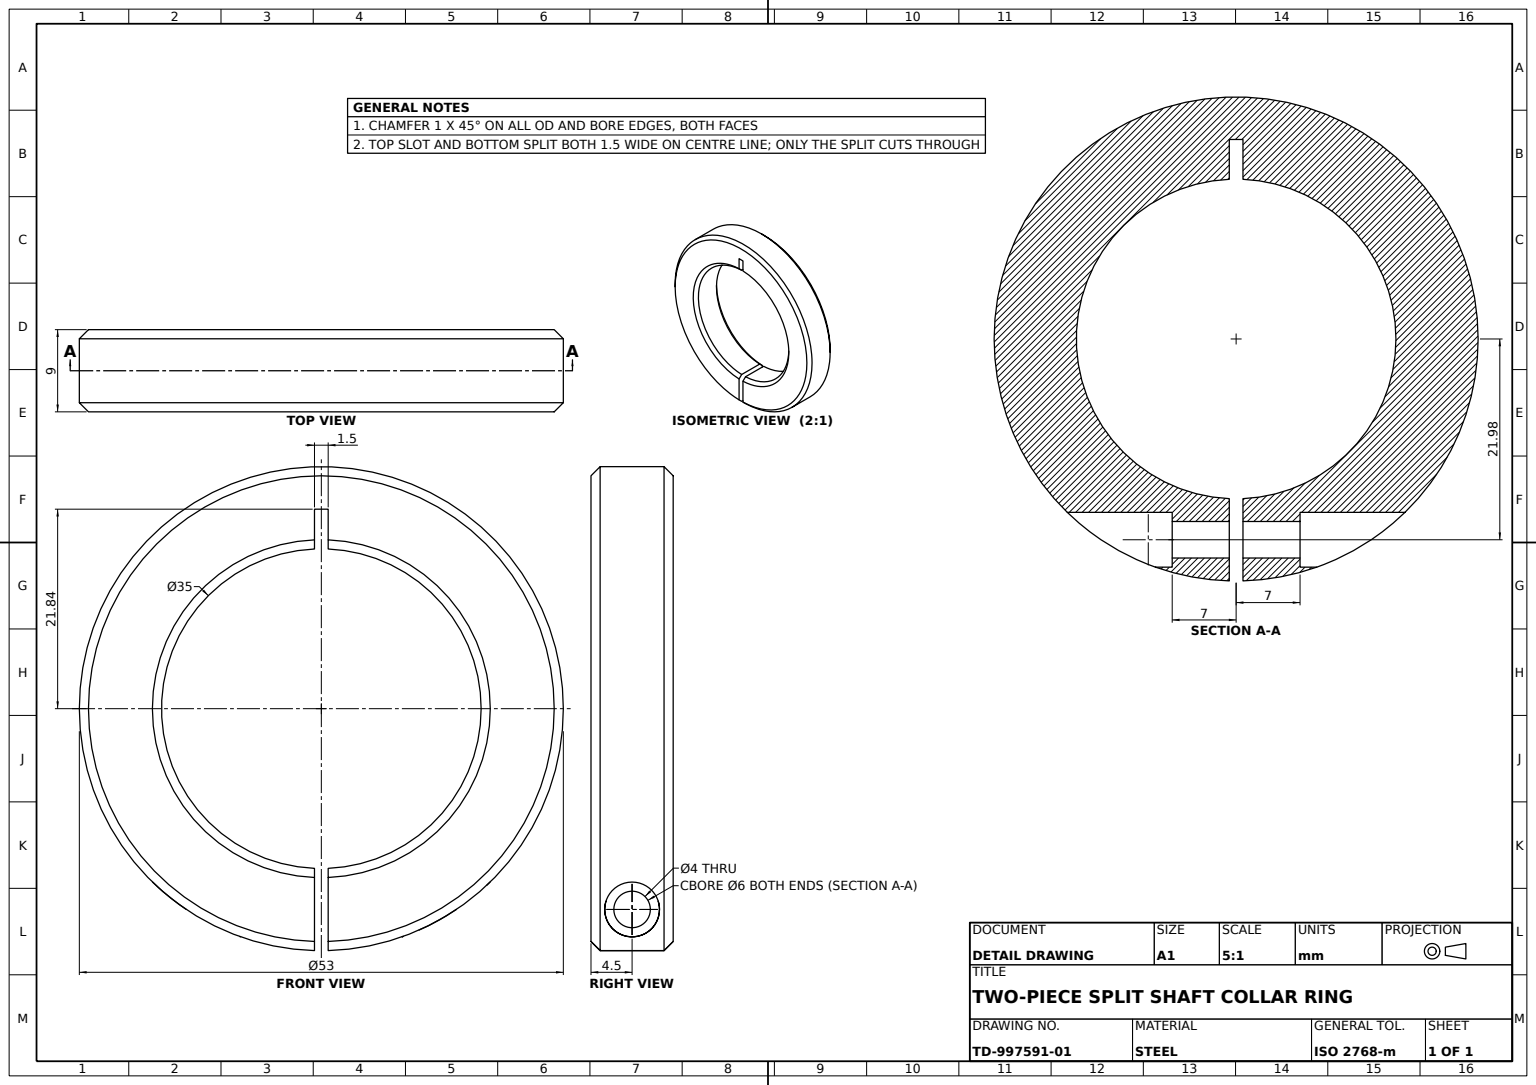
ISO-10303-21;
HEADER;
FILE_DESCRIPTION((''),'2;1');
FILE_NAME('','',(''),(''),'','','');
FILE_SCHEMA(('AUTOMOTIVE_DESIGN'));
ENDSEC;
DATA;
#1=APPLICATION_CONTEXT('');
#2=PRODUCT_CONTEXT('',#1,'mechanical');
#3=PRODUCT('','','',(#2));
#4=PRODUCT_DEFINITION_FORMATION('','',#3);
#5=PRODUCT_DEFINITION_CONTEXT('',#1,'design');
#6=PRODUCT_DEFINITION('','',#4,#5);
#7=PRODUCT_DEFINITION_SHAPE('','',#6);
#8=(LENGTH_UNIT()NAMED_UNIT(*)SI_UNIT(.MILLI.,.METRE.));
#9=(NAMED_UNIT(*)PLANE_ANGLE_UNIT()SI_UNIT($,.RADIAN.));
#10=(NAMED_UNIT(*)SI_UNIT($,.STERADIAN.)SOLID_ANGLE_UNIT());
#11=UNCERTAINTY_MEASURE_WITH_UNIT(LENGTH_MEASURE(1.E-05),#8,'distance_accuracy_value','');
#12=(GEOMETRIC_REPRESENTATION_CONTEXT(3)GLOBAL_UNCERTAINTY_ASSIGNED_CONTEXT((#11))GLOBAL_UNIT_ASSIGNED_CONTEXT((#8,#9,#10))REPRESENTATION_CONTEXT('',''));
#13=CARTESIAN_POINT('',(26.5,0.,3.5));
#14=VERTEX_POINT('',#13);
#15=CARTESIAN_POINT('',(0.75,-26.489385,3.5));
#16=VERTEX_POINT('',#15);
#17=CARTESIAN_POINT('',(0.,0.,3.5));
#18=DIRECTION('',(0.,0.,-1.));
#19=DIRECTION('',(1.,0.,0.));
#20=AXIS2_PLACEMENT_3D('',#17,#18,#19);
#21=CIRCLE('',#20,26.5);
#22=EDGE_CURVE('',#14,#16,#21,.T.);
#23=ORIENTED_EDGE('',*,*,#22,.F.);
#24=CARTESIAN_POINT('',(25.5,0.,4.5));
#25=VERTEX_POINT('',#24);
#26=DIRECTION('',(0.707106781,0.,-0.707106781));
#27=VECTOR('',#26,1000.);
#28=LINE('',#24,#27);
#29=EDGE_CURVE('',#25,#14,#28,.T.);
#30=ORIENTED_EDGE('',*,*,#29,.F.);
#31=CARTESIAN_POINT('',(0.75,-25.488968,4.5));
#32=VERTEX_POINT('',#31);
#33=CARTESIAN_POINT('',(0.,0.,4.5));
#34=DIRECTION('',(0.,0.,1.));
#35=AXIS2_PLACEMENT_3D('',#33,#34,#19);
#36=CIRCLE('',#35,25.5);
#37=EDGE_CURVE('',#32,#25,#36,.T.);
#38=ORIENTED_EDGE('',*,*,#37,.F.);
#39=CARTESIAN_POINT('',(0.75,-26.155915,3.833336));
#40=CARTESIAN_POINT('',(0.75,-25.822443,4.166669));
#41=B_SPLINE_CURVE_WITH_KNOTS('',3,(#15,#39,#40,#31),.UNSPECIFIED.,.F.,.F.,(4,4),(0.,0.001414508),.UNSPECIFIED.);
#42=EDGE_CURVE('',#16,#32,#41,.T.);
#43=ORIENTED_EDGE('',*,*,#42,.F.);
#44=EDGE_LOOP('',(#23,#30,#38,#43));
#45=FACE_OUTER_BOUND('',#44,.T.);
#46=DIRECTION('',(-1.,0.,0.));
#47=AXIS2_PLACEMENT_3D('',#33,#18,#46);
#48=CONICAL_SURFACE('',#47,25.5,0.785398163);
#49=ADVANCED_FACE('',(#45),#48,.T.);
#50=CARTESIAN_POINT('',(-17.5,0.,3.5));
#51=VERTEX_POINT('',#50);
#52=CARTESIAN_POINT('',(-17.5,0.,-3.5));
#53=VERTEX_POINT('',#52);
#54=CARTESIAN_POINT('',(-17.5,0.,4.5));
#55=VECTOR('',#18,1000.);
#56=LINE('',#54,#55);
#57=EDGE_CURVE('',#51,#53,#56,.T.);
#58=ORIENTED_EDGE('',*,*,#57,.F.);
#59=CARTESIAN_POINT('',(-0.75,-17.483921,3.5));
#60=VERTEX_POINT('',#59);
#61=AXIS2_PLACEMENT_3D('',#17,#34,#19);
#62=CIRCLE('',#61,17.5);
#63=EDGE_CURVE('',#51,#60,#62,.T.);
#64=ORIENTED_EDGE('',*,*,#63,.T.);
#65=CARTESIAN_POINT('',(-0.75,-17.483921,-3.5));
#66=VERTEX_POINT('',#65);
#67=CARTESIAN_POINT('',(-0.75,-17.483921,4.5));
#68=LINE('',#67,#55);
#69=EDGE_CURVE('',#60,#66,#68,.T.);
#70=ORIENTED_EDGE('',*,*,#69,.T.);
#71=CARTESIAN_POINT('',(0.,0.,-3.5));
#72=AXIS2_PLACEMENT_3D('',#71,#18,#19);
#73=CIRCLE('',#72,17.5);
#74=EDGE_CURVE('',#66,#53,#73,.T.);
#75=ORIENTED_EDGE('',*,*,#74,.T.);
#76=EDGE_LOOP('',(#58,#64,#70,#75));
#77=FACE_OUTER_BOUND('',#76,.T.);
#78=CYLINDRICAL_SURFACE('',#47,17.5);
#79=ADVANCED_FACE('',(#77),#78,.F.);
#80=CARTESIAN_POINT('',(-14.797203,-21.983921,3.));
#81=VERTEX_POINT('',#80);
#82=CARTESIAN_POINT('',(-14.797203,-21.983921,-3.));
#83=VERTEX_POINT('',#82);
#84=CARTESIAN_POINT('',(-14.529869,-22.163861,3.));
#85=CARTESIAN_POINT('',(-14.257232,-22.340221,2.983784));
#86=CARTESIAN_POINT('',(-13.708993,-22.680777,2.923065));
#87=CARTESIAN_POINT('',(-13.434884,-22.844118,2.878868));
#88=CARTESIAN_POINT('',(-12.612191,-23.314844,2.709228));
#89=CARTESIAN_POINT('',(-12.062916,-23.603098,2.548262));
#90=CARTESIAN_POINT('',(-11.240951,-23.999657,2.228374));
#91=CARTESIAN_POINT('',(-10.965894,-24.126449,2.107643));
#92=CARTESIAN_POINT('',(-10.428116,-24.363718,1.835525));
#93=CARTESIAN_POINT('',(-10.164897,-24.474455,1.684683));
#94=CARTESIAN_POINT('',(-9.660082,-24.678065,1.335105));
#95=CARTESIAN_POINT('',(-9.414211,-24.772349,1.13491));
#96=CARTESIAN_POINT('',(-9.110511,-24.88494,0.774549));
#97=CARTESIAN_POINT('',(-9.018443,-24.918326,0.641501));
#98=CARTESIAN_POINT('',(-8.881416,-24.967494,0.347204));
#99=CARTESIAN_POINT('',(-8.838354,-24.982664,0.184616));
#100=CARTESIAN_POINT('',(-8.833355,-24.984432,-0.059755));
#101=CARTESIAN_POINT('',(-8.841357,-24.981608,-0.14268));
#102=CARTESIAN_POINT('',(-8.875101,-24.969639,-0.303264));
#103=CARTESIAN_POINT('',(-8.900441,-24.960636,-0.380723));
#104=CARTESIAN_POINT('',(-8.997227,-24.925982,-0.606128));
#105=CARTESIAN_POINT('',(-9.085772,-24.893981,-0.740455));
#106=CARTESIAN_POINT('',(-9.287381,-24.81947,-0.988121));
#107=CARTESIAN_POINT('',(-9.400157,-24.777063,-1.100472));
#108=CARTESIAN_POINT('',(-9.634974,-24.686699,-1.30678));
#109=CARTESIAN_POINT('',(-9.758047,-24.638368,-1.401584));
#110=CARTESIAN_POINT('',(-10.138449,-24.485436,-1.668691));
#111=CARTESIAN_POINT('',(-10.405268,-24.37348,-1.822842));
#112=CARTESIAN_POINT('',(-10.942538,-24.137046,-2.096855));
#113=CARTESIAN_POINT('',(-11.215143,-24.011741,-2.217451));
#114=CARTESIAN_POINT('',(-12.040095,-23.614796,-2.541025));
#115=CARTESIAN_POINT('',(-12.602463,-23.320239,-2.706897));
#116=CARTESIAN_POINT('',(-13.431784,-22.845976,-2.878389));
#117=CARTESIAN_POINT('',(-13.706795,-22.682097,-2.922729));
#118=CARTESIAN_POINT('',(-14.254019,-22.342262,-2.983519));
#119=CARTESIAN_POINT('',(-14.527902,-22.165185,-3.));
#120=B_SPLINE_CURVE_WITH_KNOTS('',3,(#80,#84,#85,#86,#87,#88,#89,#90,#91,#92,#93,#94,#95,#96,#97,#98,#99,#100,#101,#102,#103,#104,#105,#106,#107,#108,#109,#110,#111,#112,#113,#114,#115,#116,#117,#118,#119,#82),.UNSPECIFIED.,.F.,.F.,(4,2,2,2,2,2,2,2,2,2,2,2,2,2,2,2,2,2,4),(0.012269719,0.013228684,0.014187649,0.01610558,0.017064546,0.018023511,0.018982477,0.019461959,0.019941442,0.020181183,0.020420925,0.020900407,0.02137989,0.021859373,0.022818338,0.023777304,0.025695235,0.0266542,0.027613165),.UNSPECIFIED.);
#121=EDGE_CURVE('',#81,#83,#120,.T.);
#122=ORIENTED_EDGE('',*,*,#121,.F.);
#123=CARTESIAN_POINT('',(-7.,-21.983921,3.));
#124=VERTEX_POINT('',#123);
#125=CARTESIAN_POINT('',(-32.,-21.983921,3.));
#126=VECTOR('',#19,1000.);
#127=LINE('',#125,#126);
#128=EDGE_CURVE('',#81,#124,#127,.T.);
#129=ORIENTED_EDGE('',*,*,#128,.T.);
#130=CARTESIAN_POINT('',(-7.,-21.983921,-3.));
#131=VERTEX_POINT('',#130);
#132=CARTESIAN_POINT('',(-7.,-21.983921,0.));
#133=AXIS2_PLACEMENT_3D('',#132,#19,#18);
#134=CIRCLE('',#133,3.);
#135=EDGE_CURVE('',#124,#131,#134,.T.);
#136=ORIENTED_EDGE('',*,*,#135,.T.);
#137=CARTESIAN_POINT('',(-32.,-21.983921,-3.));
#138=LINE('',#137,#126);
#139=EDGE_CURVE('',#83,#131,#138,.T.);
#140=ORIENTED_EDGE('',*,*,#139,.F.);
#141=EDGE_LOOP('',(#122,#129,#136,#140));
#142=FACE_OUTER_BOUND('',#141,.T.);
#143=CARTESIAN_POINT('',(-32.,-21.983921,0.));
#144=AXIS2_PLACEMENT_3D('',#143,#19,#18);
#145=CYLINDRICAL_SURFACE('',#144,3.);
#146=ADVANCED_FACE('',(#142),#145,.F.);
#147=CARTESIAN_POINT('',(14.797203,-21.983921,3.));
#148=VERTEX_POINT('',#147);
#149=CARTESIAN_POINT('',(7.,-21.983921,3.));
#150=VERTEX_POINT('',#149);
#151=CARTESIAN_POINT('',(32.,-21.983921,3.));
#152=VECTOR('',#46,1000.);
#153=LINE('',#151,#152);
#154=EDGE_CURVE('',#148,#150,#153,.T.);
#155=ORIENTED_EDGE('',*,*,#154,.F.);
#156=CARTESIAN_POINT('',(14.797203,-21.983921,-3.));
#157=VERTEX_POINT('',#156);
#158=CARTESIAN_POINT('',(14.255328,-22.348653,3.));
#159=CARTESIAN_POINT('',(13.708664,-22.687602,2.935579));
#160=CARTESIAN_POINT('',(12.604145,-23.319311,2.707309));
#161=CARTESIAN_POINT('',(12.042271,-23.613714,2.541794));
#162=CARTESIAN_POINT('',(11.215921,-24.011384,2.217799));
#163=CARTESIAN_POINT('',(10.942752,-24.136958,2.096985));
#164=CARTESIAN_POINT('',(10.404136,-24.373972,1.822243));
#165=CARTESIAN_POINT('',(10.137035,-24.486011,1.667748));
#166=CARTESIAN_POINT('',(9.757922,-24.638415,1.40147));
#167=CARTESIAN_POINT('',(9.634972,-24.686701,1.306797));
#168=CARTESIAN_POINT('',(9.399689,-24.777242,1.100043));
#169=CARTESIAN_POINT('',(9.286854,-24.819665,0.98749));
#170=CARTESIAN_POINT('',(9.086119,-24.893853,0.740865));
#171=CARTESIAN_POINT('',(8.996691,-24.926173,0.604627));
#172=CARTESIAN_POINT('',(8.869382,-24.971757,0.308641));
#173=CARTESIAN_POINT('',(8.832081,-24.984883,0.145601));
#174=CARTESIAN_POINT('',(8.837845,-24.982844,-0.182841));
#175=CARTESIAN_POINT('',(8.880695,-24.967748,-0.344757));
#176=CARTESIAN_POINT('',(9.016376,-24.919072,-0.637942));
#177=CARTESIAN_POINT('',(9.107598,-24.886011,-0.770787));
#178=CARTESIAN_POINT('',(9.414427,-24.772286,-1.13577));
#179=CARTESIAN_POINT('',(9.657322,-24.679165,-1.333098));
#180=CARTESIAN_POINT('',(10.165471,-24.474237,-1.685176));
#181=CARTESIAN_POINT('',(10.428836,-24.363397,-1.835876));
#182=CARTESIAN_POINT('',(10.964593,-24.127027,-2.106998));
#183=CARTESIAN_POINT('',(11.237237,-24.001422,-2.226862));
#184=CARTESIAN_POINT('',(11.788761,-23.735393,-2.441633));
#185=CARTESIAN_POINT('',(12.066283,-23.595589,-2.53578));
#186=CARTESIAN_POINT('',(12.617573,-23.305448,-2.698374));
#187=CARTESIAN_POINT('',(12.892326,-23.154642,-2.767154));
#188=CARTESIAN_POINT('',(13.713584,-22.68448,-2.936007));
#189=CARTESIAN_POINT('',(14.25693,-22.347575,-3.));
#190=B_SPLINE_CURVE_WITH_KNOTS('',3,(#147,#158,#159,#160,#161,#162,#163,#164,#165,#166,#167,#168,#169,#170,#171,#172,#173,#174,#175,#176,#177,#178,#179,#180,#181,#182,#183,#184,#185,#186,#187,#188,#189,#156),.UNSPECIFIED.,.F.,.F.,(4,2,2,2,2,2,2,2,2,2,2,2,2,2,2,2,4),(0.,0.001937428,0.003874856,0.00484357,0.005812283,0.00629664,0.006780997,0.007265354,0.007749711,0.008234068,0.008718425,0.009687139,0.010655853,0.011624567,0.012593281,0.013561995,0.015499422),.UNSPECIFIED.);
#191=EDGE_CURVE('',#148,#157,#190,.T.);
#192=ORIENTED_EDGE('',*,*,#191,.T.);
#193=CARTESIAN_POINT('',(7.,-21.983921,-3.));
#194=VERTEX_POINT('',#193);
#195=CARTESIAN_POINT('',(32.,-21.983921,-3.));
#196=LINE('',#195,#152);
#197=EDGE_CURVE('',#157,#194,#196,.T.);
#198=ORIENTED_EDGE('',*,*,#197,.T.);
#199=CARTESIAN_POINT('',(7.,-21.983921,0.));
#200=AXIS2_PLACEMENT_3D('',#199,#19,#18);
#201=CIRCLE('',#200,3.);
#202=EDGE_CURVE('',#150,#194,#201,.T.);
#203=ORIENTED_EDGE('',*,*,#202,.F.);
#204=EDGE_LOOP('',(#155,#192,#198,#203));
#205=FACE_OUTER_BOUND('',#204,.T.);
#206=CARTESIAN_POINT('',(32.,-21.983921,0.));
#207=AXIS2_PLACEMENT_3D('',#206,#46,#34);
#208=CYLINDRICAL_SURFACE('',#207,3.);
#209=ADVANCED_FACE('',(#205),#208,.F.);
#210=CARTESIAN_POINT('',(0.75,18.484791,-4.5));
#211=VERTEX_POINT('',#210);
#212=CARTESIAN_POINT('',(0.75,17.483921,-3.5));
#213=VERTEX_POINT('',#212);
#214=CARTESIAN_POINT('',(0.75,18.151176,-4.166659));
#215=CARTESIAN_POINT('',(0.75,17.817553,-3.833325));
#216=B_SPLINE_CURVE_WITH_KNOTS('',3,(#210,#214,#215,#212),.UNSPECIFIED.,.F.,.F.,(4,4),(0.,0.001414829),.UNSPECIFIED.);
#217=EDGE_CURVE('',#211,#213,#216,.T.);
#218=ORIENTED_EDGE('',*,*,#217,.F.);
#219=CARTESIAN_POINT('',(0.75,-18.484791,-4.5));
#220=VERTEX_POINT('',#219);
#221=CARTESIAN_POINT('',(0.,0.,-4.5));
#222=AXIS2_PLACEMENT_3D('',#221,#34,#19);
#223=CIRCLE('',#222,18.5);
#224=EDGE_CURVE('',#220,#211,#223,.T.);
#225=ORIENTED_EDGE('',*,*,#224,.F.);
#226=CARTESIAN_POINT('',(0.75,-17.483921,-3.5));
#227=VERTEX_POINT('',#226);
#228=CARTESIAN_POINT('',(0.75,-17.817553,-3.833325));
#229=CARTESIAN_POINT('',(0.75,-18.151176,-4.166659));
#230=B_SPLINE_CURVE_WITH_KNOTS('',3,(#226,#228,#229,#219),.UNSPECIFIED.,.F.,.F.,(4,4),(0.,0.001414829),.UNSPECIFIED.);
#231=EDGE_CURVE('',#227,#220,#230,.T.);
#232=ORIENTED_EDGE('',*,*,#231,.F.);
#233=EDGE_CURVE('',#213,#227,#73,.T.);
#234=ORIENTED_EDGE('',*,*,#233,.F.);
#235=EDGE_LOOP('',(#218,#225,#232,#234));
#236=FACE_OUTER_BOUND('',#235,.T.);
#237=AXIS2_PLACEMENT_3D('',#71,#18,#46);
#238=CONICAL_SURFACE('',#237,17.5,0.785398163);
#239=ADVANCED_FACE('',(#236),#238,.F.);
#240=ORIENTED_EDGE('',*,*,#29,.T.);
#241=CARTESIAN_POINT('',(-26.5,0.,3.5));
#242=VERTEX_POINT('',#241);
#243=EDGE_CURVE('',#242,#14,#21,.T.);
#244=ORIENTED_EDGE('',*,*,#243,.F.);
#245=CARTESIAN_POINT('',(-25.5,0.,4.5));
#246=VERTEX_POINT('',#245);
#247=DIRECTION('',(-0.707106781,0.,-0.707106781));
#248=VECTOR('',#247,1000.);
#249=LINE('',#245,#248);
#250=EDGE_CURVE('',#246,#242,#249,.T.);
#251=ORIENTED_EDGE('',*,*,#250,.F.);
#252=EDGE_CURVE('',#25,#246,#36,.T.);
#253=ORIENTED_EDGE('',*,*,#252,.F.);
#254=EDGE_LOOP('',(#240,#244,#251,#253));
#255=FACE_OUTER_BOUND('',#254,.T.);
#256=ADVANCED_FACE('',(#255),#48,.T.);
#257=CARTESIAN_POINT('',(-0.75,18.484791,-4.5));
#258=VERTEX_POINT('',#257);
#259=CARTESIAN_POINT('',(-18.5,0.,-4.5));
#260=VERTEX_POINT('',#259);
#261=EDGE_CURVE('',#258,#260,#223,.T.);
#262=ORIENTED_EDGE('',*,*,#261,.F.);
#263=CARTESIAN_POINT('',(-0.75,17.483921,-3.5));
#264=VERTEX_POINT('',#263);
#265=CARTESIAN_POINT('',(-0.75,17.817553,-3.833325));
#266=CARTESIAN_POINT('',(-0.75,18.151176,-4.166659));
#267=B_SPLINE_CURVE_WITH_KNOTS('',3,(#263,#265,#266,#257),.UNSPECIFIED.,.F.,.F.,(4,4),(0.,0.001414829),.UNSPECIFIED.);
#268=EDGE_CURVE('',#264,#258,#267,.T.);
#269=ORIENTED_EDGE('',*,*,#268,.F.);
#270=EDGE_CURVE('',#53,#264,#73,.T.);
#271=ORIENTED_EDGE('',*,*,#270,.F.);
#272=LINE('',#52,#248);
#273=EDGE_CURVE('',#53,#260,#272,.T.);
#274=ORIENTED_EDGE('',*,*,#273,.T.);
#275=EDGE_LOOP('',(#262,#269,#271,#274));
#276=FACE_OUTER_BOUND('',#275,.T.);
#277=ADVANCED_FACE('',(#276),#238,.F.);
#278=ORIENTED_EDGE('',*,*,#74,.F.);
#279=CARTESIAN_POINT('',(-0.75,-18.484791,-4.5));
#280=VERTEX_POINT('',#279);
#281=CARTESIAN_POINT('',(-0.75,-18.151176,-4.166659));
#282=CARTESIAN_POINT('',(-0.75,-17.817553,-3.833325));
#283=B_SPLINE_CURVE_WITH_KNOTS('',3,(#279,#281,#282,#65),.UNSPECIFIED.,.F.,.F.,(4,4),(0.,0.001414829),.UNSPECIFIED.);
#284=EDGE_CURVE('',#280,#66,#283,.T.);
#285=ORIENTED_EDGE('',*,*,#284,.F.);
#286=EDGE_CURVE('',#260,#280,#223,.T.);
#287=ORIENTED_EDGE('',*,*,#286,.F.);
#288=ORIENTED_EDGE('',*,*,#273,.F.);
#289=EDGE_LOOP('',(#278,#285,#287,#288));
#290=FACE_OUTER_BOUND('',#289,.T.);
#291=ADVANCED_FACE('',(#290),#238,.F.);
#292=CARTESIAN_POINT('',(-26.5,0.,-3.5));
#293=VERTEX_POINT('',#292);
#294=CARTESIAN_POINT('',(-0.75,-26.489385,-3.5));
#295=VERTEX_POINT('',#294);
#296=AXIS2_PLACEMENT_3D('',#71,#34,#19);
#297=CIRCLE('',#296,26.5);
#298=EDGE_CURVE('',#293,#295,#297,.T.);
#299=ORIENTED_EDGE('',*,*,#298,.F.);
#300=CARTESIAN_POINT('',(-25.5,0.,-4.5));
#301=VERTEX_POINT('',#300);
#302=DIRECTION('',(-0.707106781,0.,0.707106781));
#303=VECTOR('',#302,1000.);
#304=LINE('',#292,#303);
#305=EDGE_CURVE('',#301,#293,#304,.T.);
#306=ORIENTED_EDGE('',*,*,#305,.F.);
#307=CARTESIAN_POINT('',(-0.75,-25.488968,-4.5));
#308=VERTEX_POINT('',#307);
#309=AXIS2_PLACEMENT_3D('',#221,#18,#19);
#310=CIRCLE('',#309,25.5);
#311=EDGE_CURVE('',#308,#301,#310,.T.);
#312=ORIENTED_EDGE('',*,*,#311,.F.);
#313=CARTESIAN_POINT('',(-0.75,-26.155915,-3.833336));
#314=CARTESIAN_POINT('',(-0.75,-25.822443,-4.166669));
#315=B_SPLINE_CURVE_WITH_KNOTS('',3,(#294,#313,#314,#307),.UNSPECIFIED.,.F.,.F.,(4,4),(0.,0.001414508),.UNSPECIFIED.);
#316=EDGE_CURVE('',#295,#308,#315,.T.);
#317=ORIENTED_EDGE('',*,*,#316,.F.);
#318=EDGE_LOOP('',(#299,#306,#312,#317));
#319=FACE_OUTER_BOUND('',#318,.T.);
#320=CONICAL_SURFACE('',#296,26.5,0.785398163);
#321=ADVANCED_FACE('',(#319),#320,.T.);
#322=CARTESIAN_POINT('',(0.75,-21.983921,2.));
#323=VERTEX_POINT('',#322);
#324=CARTESIAN_POINT('',(7.,-21.983921,2.));
#325=VERTEX_POINT('',#324);
#326=CARTESIAN_POINT('',(-26.5,-21.983921,2.));
#327=LINE('',#326,#126);
#328=EDGE_CURVE('',#323,#325,#327,.T.);
#329=ORIENTED_EDGE('',*,*,#328,.F.);
#330=CARTESIAN_POINT('',(0.75,-21.983921,-2.));
#331=VERTEX_POINT('',#330);
#332=CARTESIAN_POINT('',(0.75,-21.983921,0.));
#333=AXIS2_PLACEMENT_3D('',#332,#19,#18);
#334=CIRCLE('',#333,2.);
#335=EDGE_CURVE('',#331,#323,#334,.T.);
#336=ORIENTED_EDGE('',*,*,#335,.F.);
#337=CARTESIAN_POINT('',(7.,-21.983921,-2.));
#338=VERTEX_POINT('',#337);
#339=CARTESIAN_POINT('',(-26.5,-21.983921,-2.));
#340=LINE('',#339,#126);
#341=EDGE_CURVE('',#331,#338,#340,.T.);
#342=ORIENTED_EDGE('',*,*,#341,.T.);
#343=AXIS2_PLACEMENT_3D('',#199,#46,#18);
#344=CIRCLE('',#343,2.);
#345=EDGE_CURVE('',#325,#338,#344,.T.);
#346=ORIENTED_EDGE('',*,*,#345,.F.);
#347=EDGE_LOOP('',(#329,#336,#342,#346));
#348=FACE_OUTER_BOUND('',#347,.T.);
#349=CARTESIAN_POINT('',(-26.5,-21.983921,0.));
#350=AXIS2_PLACEMENT_3D('',#349,#19,#18);
#351=CYLINDRICAL_SURFACE('',#350,2.);
#352=ADVANCED_FACE('',(#348),#351,.F.);
#353=CARTESIAN_POINT('',(0.75,21.843891,-4.5));
#354=VERTEX_POINT('',#353);
#355=DIRECTION('',(0.,-1.,0.));
#356=VECTOR('',#355,1000.);
#357=LINE('',#353,#356);
#358=EDGE_CURVE('',#354,#211,#357,.T.);
#359=ORIENTED_EDGE('',*,*,#358,.F.);
#360=CARTESIAN_POINT('',(-0.75,21.843891,-4.5));
#361=VERTEX_POINT('',#360);
#362=LINE('',#360,#126);
#363=EDGE_CURVE('',#361,#354,#362,.T.);
#364=ORIENTED_EDGE('',*,*,#363,.F.);
#365=CARTESIAN_POINT('',(-0.75,17.483921,-4.5));
#366=DIRECTION('',(0.,1.,0.));
#367=VECTOR('',#366,1000.);
#368=LINE('',#365,#367);
#369=EDGE_CURVE('',#258,#361,#368,.T.);
#370=ORIENTED_EDGE('',*,*,#369,.F.);
#371=ORIENTED_EDGE('',*,*,#261,.T.);
#372=ORIENTED_EDGE('',*,*,#286,.T.);
#373=CARTESIAN_POINT('',(-0.75,-17.483921,-4.5));
#374=LINE('',#373,#367);
#375=EDGE_CURVE('',#308,#280,#374,.T.);
#376=ORIENTED_EDGE('',*,*,#375,.F.);
#377=ORIENTED_EDGE('',*,*,#311,.T.);
#378=CARTESIAN_POINT('',(25.5,0.,-4.5));
#379=VERTEX_POINT('',#378);
#380=EDGE_CURVE('',#301,#379,#310,.T.);
#381=ORIENTED_EDGE('',*,*,#380,.T.);
#382=CARTESIAN_POINT('',(0.75,-25.488968,-4.5));
#383=VERTEX_POINT('',#382);
#384=EDGE_CURVE('',#379,#383,#310,.T.);
#385=ORIENTED_EDGE('',*,*,#384,.T.);
#386=CARTESIAN_POINT('',(0.75,-26.489385,-4.5));
#387=LINE('',#386,#356);
#388=EDGE_CURVE('',#220,#383,#387,.T.);
#389=ORIENTED_EDGE('',*,*,#388,.F.);
#390=ORIENTED_EDGE('',*,*,#224,.T.);
#391=EDGE_LOOP('',(#359,#364,#370,#371,#372,#376,#377,#381,#385,#389,#390));
#392=FACE_OUTER_BOUND('',#391,.T.);
#393=PLANE('',#222);
#394=ADVANCED_FACE('',(#392),#393,.F.);
#395=CARTESIAN_POINT('',(0.75,-17.483921,3.5));
#396=VERTEX_POINT('',#395);
#397=CARTESIAN_POINT('',(0.75,-17.483921,4.5));
#398=LINE('',#397,#55);
#399=EDGE_CURVE('',#396,#227,#398,.T.);
#400=ORIENTED_EDGE('',*,*,#399,.T.);
#401=ORIENTED_EDGE('',*,*,#231,.T.);
#402=ORIENTED_EDGE('',*,*,#388,.T.);
#403=CARTESIAN_POINT('',(0.75,-26.489385,-3.5));
#404=VERTEX_POINT('',#403);
#405=CARTESIAN_POINT('',(0.75,-25.822443,-4.166669));
#406=CARTESIAN_POINT('',(0.75,-26.155915,-3.833336));
#407=B_SPLINE_CURVE_WITH_KNOTS('',3,(#382,#405,#406,#403),.UNSPECIFIED.,.F.,.F.,(4,4),(0.,0.001414508),.UNSPECIFIED.);
#408=EDGE_CURVE('',#383,#404,#407,.T.);
#409=ORIENTED_EDGE('',*,*,#408,.T.);
#410=CARTESIAN_POINT('',(0.75,-26.489385,4.5));
#411=LINE('',#410,#55);
#412=EDGE_CURVE('',#16,#404,#411,.T.);
#413=ORIENTED_EDGE('',*,*,#412,.F.);
#414=ORIENTED_EDGE('',*,*,#42,.T.);
#415=CARTESIAN_POINT('',(0.75,-18.484791,4.5));
#416=VERTEX_POINT('',#415);
#417=LINE('',#410,#356);
#418=EDGE_CURVE('',#416,#32,#417,.T.);
#419=ORIENTED_EDGE('',*,*,#418,.F.);
#420=CARTESIAN_POINT('',(0.75,-18.151176,4.166659));
#421=CARTESIAN_POINT('',(0.75,-17.817553,3.833325));
#422=B_SPLINE_CURVE_WITH_KNOTS('',3,(#415,#420,#421,#395),.UNSPECIFIED.,.F.,.F.,(4,4),(0.,0.001414829),.UNSPECIFIED.);
#423=EDGE_CURVE('',#416,#396,#422,.T.);
#424=ORIENTED_EDGE('',*,*,#423,.T.);
#425=EDGE_LOOP('',(#400,#401,#402,#409,#413,#414,#419,#424));
#426=FACE_OUTER_BOUND('',#425,.T.);
#427=ORIENTED_EDGE('',*,*,#335,.T.);
#428=EDGE_CURVE('',#323,#331,#334,.T.);
#429=ORIENTED_EDGE('',*,*,#428,.T.);
#430=EDGE_LOOP('',(#427,#429));
#431=FACE_BOUND('',#430,.T.);
#432=AXIS2_PLACEMENT_3D('',#410,#19,#18);
#433=PLANE('',#432);
#434=ADVANCED_FACE('',(#426,#431),#433,.F.);
#435=CARTESIAN_POINT('',(0.75,17.483921,3.5));
#436=VERTEX_POINT('',#435);
#437=CARTESIAN_POINT('',(0.75,17.483921,4.5));
#438=LINE('',#437,#55);
#439=EDGE_CURVE('',#436,#213,#438,.T.);
#440=ORIENTED_EDGE('',*,*,#439,.T.);
#441=ORIENTED_EDGE('',*,*,#233,.T.);
#442=ORIENTED_EDGE('',*,*,#399,.F.);
#443=CARTESIAN_POINT('',(17.5,0.,3.5));
#444=VERTEX_POINT('',#443);
#445=EDGE_CURVE('',#396,#444,#62,.T.);
#446=ORIENTED_EDGE('',*,*,#445,.T.);
#447=EDGE_CURVE('',#444,#436,#62,.T.);
#448=ORIENTED_EDGE('',*,*,#447,.T.);
#449=EDGE_LOOP('',(#440,#441,#442,#446,#448));
#450=FACE_OUTER_BOUND('',#449,.T.);
#451=ADVANCED_FACE('',(#450),#78,.F.);
#452=CARTESIAN_POINT('',(-7.,-21.983921,-2.));
#453=VERTEX_POINT('',#452);
#454=CARTESIAN_POINT('',(-0.75,-21.983921,-2.));
#455=VERTEX_POINT('',#454);
#456=EDGE_CURVE('',#453,#455,#340,.T.);
#457=ORIENTED_EDGE('',*,*,#456,.F.);
#458=CARTESIAN_POINT('',(-7.,-21.983921,2.));
#459=VERTEX_POINT('',#458);
#460=AXIS2_PLACEMENT_3D('',#132,#19,#34);
#461=CIRCLE('',#460,2.);
#462=EDGE_CURVE('',#459,#453,#461,.T.);
#463=ORIENTED_EDGE('',*,*,#462,.F.);
#464=CARTESIAN_POINT('',(-0.75,-21.983921,2.));
#465=VERTEX_POINT('',#464);
#466=EDGE_CURVE('',#459,#465,#327,.T.);
#467=ORIENTED_EDGE('',*,*,#466,.T.);
#468=CARTESIAN_POINT('',(-0.75,-21.983921,0.));
#469=AXIS2_PLACEMENT_3D('',#468,#46,#34);
#470=CIRCLE('',#469,2.);
#471=EDGE_CURVE('',#455,#465,#470,.T.);
#472=ORIENTED_EDGE('',*,*,#471,.F.);
#473=EDGE_LOOP('',(#457,#463,#467,#472));
#474=FACE_OUTER_BOUND('',#473,.T.);
#475=ADVANCED_FACE('',(#474),#351,.F.);
#476=CARTESIAN_POINT('',(0.75,18.484791,4.5));
#477=VERTEX_POINT('',#476);
#478=CARTESIAN_POINT('',(0.75,17.817553,3.833325));
#479=CARTESIAN_POINT('',(0.75,18.151176,4.166659));
#480=B_SPLINE_CURVE_WITH_KNOTS('',3,(#435,#478,#479,#476),.UNSPECIFIED.,.F.,.F.,(4,4),(0.,0.001414829),.UNSPECIFIED.);
#481=EDGE_CURVE('',#436,#477,#480,.T.);
#482=ORIENTED_EDGE('',*,*,#481,.F.);
#483=ORIENTED_EDGE('',*,*,#447,.F.);
#484=CARTESIAN_POINT('',(18.5,0.,4.5));
#485=VERTEX_POINT('',#484);
#486=DIRECTION('',(0.707106781,0.,0.707106781));
#487=VECTOR('',#486,1000.);
#488=LINE('',#484,#487);
#489=EDGE_CURVE('',#444,#485,#488,.T.);
#490=ORIENTED_EDGE('',*,*,#489,.T.);
#491=AXIS2_PLACEMENT_3D('',#33,#18,#19);
#492=CIRCLE('',#491,18.5);
#493=EDGE_CURVE('',#477,#485,#492,.T.);
#494=ORIENTED_EDGE('',*,*,#493,.F.);
#495=EDGE_LOOP('',(#482,#483,#490,#494));
#496=FACE_OUTER_BOUND('',#495,.T.);
#497=CONICAL_SURFACE('',#35,18.5,0.785398163);
#498=ADVANCED_FACE('',(#496),#497,.F.);
#499=CARTESIAN_POINT('',(26.5,0.,-3.5));
#500=VERTEX_POINT('',#499);
#501=EDGE_CURVE('',#404,#500,#297,.T.);
#502=ORIENTED_EDGE('',*,*,#501,.F.);
#503=ORIENTED_EDGE('',*,*,#408,.F.);
#504=ORIENTED_EDGE('',*,*,#384,.F.);
#505=LINE('',#499,#487);
#506=EDGE_CURVE('',#379,#500,#505,.T.);
#507=ORIENTED_EDGE('',*,*,#506,.T.);
#508=EDGE_LOOP('',(#502,#503,#504,#507));
#509=FACE_OUTER_BOUND('',#508,.T.);
#510=ADVANCED_FACE('',(#509),#320,.T.);
#511=ORIENTED_EDGE('',*,*,#358,.T.);
#512=ORIENTED_EDGE('',*,*,#217,.T.);
#513=ORIENTED_EDGE('',*,*,#439,.F.);
#514=ORIENTED_EDGE('',*,*,#481,.T.);
#515=CARTESIAN_POINT('',(0.75,21.843891,4.5));
#516=VERTEX_POINT('',#515);
#517=LINE('',#515,#356);
#518=EDGE_CURVE('',#516,#477,#517,.T.);
#519=ORIENTED_EDGE('',*,*,#518,.F.);
#520=LINE('',#515,#55);
#521=EDGE_CURVE('',#516,#354,#520,.T.);
#522=ORIENTED_EDGE('',*,*,#521,.T.);
#523=EDGE_LOOP('',(#511,#512,#513,#514,#519,#522));
#524=FACE_OUTER_BOUND('',#523,.T.);
#525=AXIS2_PLACEMENT_3D('',#515,#19,#366);
#526=PLANE('',#525);
#527=ADVANCED_FACE('',(#524),#526,.F.);
#528=CARTESIAN_POINT('',(-0.75,17.483921,3.5));
#529=VERTEX_POINT('',#528);
#530=CARTESIAN_POINT('',(-0.75,17.483921,4.5));
#531=LINE('',#530,#55);
#532=EDGE_CURVE('',#529,#264,#531,.T.);
#533=ORIENTED_EDGE('',*,*,#532,.F.);
#534=EDGE_CURVE('',#529,#51,#62,.T.);
#535=ORIENTED_EDGE('',*,*,#534,.T.);
#536=ORIENTED_EDGE('',*,*,#57,.T.);
#537=ORIENTED_EDGE('',*,*,#270,.T.);
#538=EDGE_LOOP('',(#533,#535,#536,#537));
#539=FACE_OUTER_BOUND('',#538,.T.);
#540=ADVANCED_FACE('',(#539),#78,.F.);
#541=ORIENTED_EDGE('',*,*,#135,.F.);
#542=EDGE_CURVE('',#131,#124,#134,.T.);
#543=ORIENTED_EDGE('',*,*,#542,.F.);
#544=EDGE_LOOP('',(#541,#543));
#545=FACE_OUTER_BOUND('',#544,.T.);
#546=ORIENTED_EDGE('',*,*,#462,.T.);
#547=EDGE_CURVE('',#453,#459,#461,.T.);
#548=ORIENTED_EDGE('',*,*,#547,.T.);
#549=EDGE_LOOP('',(#546,#548));
#550=FACE_BOUND('',#549,.T.);
#551=AXIS2_PLACEMENT_3D('',#132,#46,#18);
#552=PLANE('',#551);
#553=ADVANCED_FACE('',(#545,#550),#552,.T.);
#554=ORIENTED_EDGE('',*,*,#456,.T.);
#555=EDGE_CURVE('',#465,#455,#470,.T.);
#556=ORIENTED_EDGE('',*,*,#555,.F.);
#557=ORIENTED_EDGE('',*,*,#466,.F.);
#558=ORIENTED_EDGE('',*,*,#547,.F.);
#559=EDGE_LOOP('',(#554,#556,#557,#558));
#560=FACE_OUTER_BOUND('',#559,.T.);
#561=ADVANCED_FACE('',(#560),#351,.F.);
#562=ORIENTED_EDGE('',*,*,#489,.F.);
#563=ORIENTED_EDGE('',*,*,#445,.F.);
#564=ORIENTED_EDGE('',*,*,#423,.F.);
#565=EDGE_CURVE('',#485,#416,#492,.T.);
#566=ORIENTED_EDGE('',*,*,#565,.F.);
#567=EDGE_LOOP('',(#562,#563,#564,#566));
#568=FACE_OUTER_BOUND('',#567,.T.);
#569=ADVANCED_FACE('',(#568),#497,.F.);
#570=EDGE_CURVE('',#338,#325,#344,.T.);
#571=ORIENTED_EDGE('',*,*,#570,.F.);
#572=ORIENTED_EDGE('',*,*,#341,.F.);
#573=ORIENTED_EDGE('',*,*,#428,.F.);
#574=ORIENTED_EDGE('',*,*,#328,.T.);
#575=EDGE_LOOP('',(#571,#572,#573,#574));
#576=FACE_OUTER_BOUND('',#575,.T.);
#577=ADVANCED_FACE('',(#576),#351,.F.);
#578=ORIENTED_EDGE('',*,*,#363,.T.);
#579=ORIENTED_EDGE('',*,*,#521,.F.);
#580=CARTESIAN_POINT('',(-0.75,21.843891,4.5));
#581=VERTEX_POINT('',#580);
#582=LINE('',#580,#126);
#583=EDGE_CURVE('',#581,#516,#582,.T.);
#584=ORIENTED_EDGE('',*,*,#583,.F.);
#585=LINE('',#580,#55);
#586=EDGE_CURVE('',#581,#361,#585,.T.);
#587=ORIENTED_EDGE('',*,*,#586,.T.);
#588=EDGE_LOOP('',(#578,#579,#584,#587));
#589=FACE_OUTER_BOUND('',#588,.T.);
#590=AXIS2_PLACEMENT_3D('',#580,#366,#34);
#591=PLANE('',#590);
#592=ADVANCED_FACE('',(#589),#591,.F.);
#593=CARTESIAN_POINT('',(-0.75,-25.488968,4.5));
#594=VERTEX_POINT('',#593);
#595=CARTESIAN_POINT('',(-0.75,-26.489385,3.5));
#596=VERTEX_POINT('',#595);
#597=CARTESIAN_POINT('',(-0.75,-25.822443,4.166669));
#598=CARTESIAN_POINT('',(-0.75,-26.155915,3.833336));
#599=B_SPLINE_CURVE_WITH_KNOTS('',3,(#593,#597,#598,#595),.UNSPECIFIED.,.F.,.F.,(4,4),(0.,0.001414508),.UNSPECIFIED.);
#600=EDGE_CURVE('',#594,#596,#599,.T.);
#601=ORIENTED_EDGE('',*,*,#600,.F.);
#602=EDGE_CURVE('',#246,#594,#36,.T.);
#603=ORIENTED_EDGE('',*,*,#602,.F.);
#604=ORIENTED_EDGE('',*,*,#250,.T.);
#605=EDGE_CURVE('',#596,#242,#21,.T.);
#606=ORIENTED_EDGE('',*,*,#605,.F.);
#607=EDGE_LOOP('',(#601,#603,#604,#606));
#608=FACE_OUTER_BOUND('',#607,.T.);
#609=ADVANCED_FACE('',(#608),#48,.T.);
#610=CARTESIAN_POINT('',(-0.75,18.484791,4.5));
#611=VERTEX_POINT('',#610);
#612=LINE('',#530,#367);
#613=EDGE_CURVE('',#611,#581,#612,.T.);
#614=ORIENTED_EDGE('',*,*,#613,.T.);
#615=ORIENTED_EDGE('',*,*,#583,.T.);
#616=ORIENTED_EDGE('',*,*,#518,.T.);
#617=ORIENTED_EDGE('',*,*,#493,.T.);
#618=ORIENTED_EDGE('',*,*,#565,.T.);
#619=ORIENTED_EDGE('',*,*,#418,.T.);
#620=ORIENTED_EDGE('',*,*,#37,.T.);
#621=ORIENTED_EDGE('',*,*,#252,.T.);
#622=ORIENTED_EDGE('',*,*,#602,.T.);
#623=CARTESIAN_POINT('',(-0.75,-18.484791,4.5));
#624=VERTEX_POINT('',#623);
#625=LINE('',#67,#367);
#626=EDGE_CURVE('',#594,#624,#625,.T.);
#627=ORIENTED_EDGE('',*,*,#626,.T.);
#628=EDGE_CURVE('',#624,#611,#492,.T.);
#629=ORIENTED_EDGE('',*,*,#628,.T.);
#630=EDGE_LOOP('',(#614,#615,#616,#617,#618,#619,#620,#621,#622,#627,#629));
#631=FACE_OUTER_BOUND('',#630,.T.);
#632=PLANE('',#35);
#633=ADVANCED_FACE('',(#631),#632,.T.);
#634=CARTESIAN_POINT('',(15.228297,-21.693755,-3.));
#635=CARTESIAN_POINT('',(15.646514,-21.393792,-2.958986));
#636=CARTESIAN_POINT('',(16.252479,-20.932544,-2.81435));
#637=CARTESIAN_POINT('',(16.452169,-20.775875,-2.751523));
#638=CARTESIAN_POINT('',(16.836117,-20.465973,-2.59347));
#639=CARTESIAN_POINT('',(17.020572,-20.312648,-2.498512));
#640=CARTESIAN_POINT('',(17.372704,-20.012313,-2.269026));
#641=CARTESIAN_POINT('',(17.541978,-19.863822,-2.132794));
#642=CARTESIAN_POINT('',(17.848657,-19.588718,-1.818414));
#643=CARTESIAN_POINT('',(17.987744,-19.460668,-1.639309));
#644=CARTESIAN_POINT('',(18.225619,-19.23807,-1.230627));
#645=CARTESIAN_POINT('',(18.320994,-19.146797,-1.007541));
#646=CARTESIAN_POINT('',(18.454804,-19.017856,-0.516595));
#647=CARTESIAN_POINT('',(18.489342,-18.984052,-0.263279));
#648=CARTESIAN_POINT('',(18.48961,-18.983791,0.260294));
#649=CARTESIAN_POINT('',(18.454731,-19.017928,0.517084));
#650=CARTESIAN_POINT('',(18.320724,-19.147055,1.008308));
#651=CARTESIAN_POINT('',(18.224381,-19.239245,1.233245));
#652=CARTESIAN_POINT('',(17.986062,-19.462225,1.641702));
#653=CARTESIAN_POINT('',(17.847902,-19.589412,1.819378));
#654=CARTESIAN_POINT('',(17.54037,-19.865248,2.134252));
#655=CARTESIAN_POINT('',(17.371414,-20.01343,2.269973));
#656=CARTESIAN_POINT('',(17.01965,-20.313418,2.499006));
#657=CARTESIAN_POINT('',(16.835087,-20.466826,2.59399));
#658=CARTESIAN_POINT('',(16.450303,-20.777359,2.752194));
#659=CARTESIAN_POINT('',(16.251029,-20.933664,2.814753));
#660=CARTESIAN_POINT('',(15.645995,-21.394153,2.958997));
#661=CARTESIAN_POINT('',(15.229575,-21.692895,3.));
#662=B_SPLINE_CURVE_WITH_KNOTS('',3,(#156,#634,#635,#636,#637,#638,#639,#640,#641,#642,#643,#644,#645,#646,#647,#648,#649,#650,#651,#652,#653,#654,#655,#656,#657,#658,#659,#660,#661,#147),.UNSPECIFIED.,.F.,.F.,(4,2,2,2,2,2,2,2,2,2,2,2,2,2,4),(0.015499422,0.017045334,0.01781829,0.018591246,0.019364202,0.020137157,0.020910113,0.021683069,0.022456025,0.023228981,0.024001937,0.024774892,0.025547848,0.026320804,0.027866716),.UNSPECIFIED.);
#663=EDGE_CURVE('',#157,#148,#662,.T.);
#664=ORIENTED_EDGE('',*,*,#663,.F.);
#665=ORIENTED_EDGE('',*,*,#191,.F.);
#666=EDGE_LOOP('',(#664,#665));
#667=FACE_BOUND('',#666,.T.);
#668=ORIENTED_EDGE('',*,*,#501,.T.);
#669=CARTESIAN_POINT('',(26.5,0.,4.5));
#670=LINE('',#669,#55);
#671=EDGE_CURVE('',#14,#500,#670,.T.);
#672=ORIENTED_EDGE('',*,*,#671,.F.);
#673=ORIENTED_EDGE('',*,*,#22,.T.);
#674=ORIENTED_EDGE('',*,*,#412,.T.);
#675=EDGE_LOOP('',(#668,#672,#673,#674));
#676=FACE_OUTER_BOUND('',#675,.T.);
#677=CYLINDRICAL_SURFACE('',#47,26.5);
#678=ADVANCED_FACE('',(#667,#676),#677,.T.);
#679=ORIENTED_EDGE('',*,*,#570,.T.);
#680=ORIENTED_EDGE('',*,*,#345,.T.);
#681=EDGE_LOOP('',(#679,#680));
#682=FACE_BOUND('',#681,.T.);
#683=ORIENTED_EDGE('',*,*,#202,.T.);
#684=EDGE_CURVE('',#194,#150,#201,.T.);
#685=ORIENTED_EDGE('',*,*,#684,.T.);
#686=EDGE_LOOP('',(#683,#685));
#687=FACE_OUTER_BOUND('',#686,.T.);
#688=PLANE('',#200);
#689=ADVANCED_FACE('',(#682,#687),#688,.T.);
#690=ORIENTED_EDGE('',*,*,#375,.T.);
#691=ORIENTED_EDGE('',*,*,#284,.T.);
#692=ORIENTED_EDGE('',*,*,#69,.F.);
#693=CARTESIAN_POINT('',(-0.75,-17.817553,3.833325));
#694=CARTESIAN_POINT('',(-0.75,-18.151176,4.166659));
#695=B_SPLINE_CURVE_WITH_KNOTS('',3,(#59,#693,#694,#623),.UNSPECIFIED.,.F.,.F.,(4,4),(0.,0.001414829),.UNSPECIFIED.);
#696=EDGE_CURVE('',#60,#624,#695,.T.);
#697=ORIENTED_EDGE('',*,*,#696,.T.);
#698=ORIENTED_EDGE('',*,*,#626,.F.);
#699=ORIENTED_EDGE('',*,*,#600,.T.);
#700=CARTESIAN_POINT('',(-0.75,-26.489385,4.5));
#701=LINE('',#700,#55);
#702=EDGE_CURVE('',#596,#295,#701,.T.);
#703=ORIENTED_EDGE('',*,*,#702,.T.);
#704=ORIENTED_EDGE('',*,*,#316,.T.);
#705=EDGE_LOOP('',(#690,#691,#692,#697,#698,#699,#703,#704));
#706=FACE_OUTER_BOUND('',#705,.T.);
#707=ORIENTED_EDGE('',*,*,#471,.T.);
#708=ORIENTED_EDGE('',*,*,#555,.T.);
#709=EDGE_LOOP('',(#707,#708));
#710=FACE_BOUND('',#709,.T.);
#711=AXIS2_PLACEMENT_3D('',#67,#46,#34);
#712=PLANE('',#711);
#713=ADVANCED_FACE('',(#706,#710),#712,.F.);
#714=ORIENTED_EDGE('',*,*,#139,.T.);
#715=ORIENTED_EDGE('',*,*,#542,.T.);
#716=ORIENTED_EDGE('',*,*,#128,.F.);
#717=CARTESIAN_POINT('',(-15.227906,-21.694018,-3.));
#718=CARTESIAN_POINT('',(-15.643668,-21.395751,-2.958984));
#719=CARTESIAN_POINT('',(-16.243559,-20.939434,-2.816812));
#720=CARTESIAN_POINT('',(-16.439546,-20.785859,-2.755832));
#721=CARTESIAN_POINT('',(-16.822892,-20.476839,-2.599744));
#722=CARTESIAN_POINT('',(-17.01138,-20.320363,-2.503705));
#723=CARTESIAN_POINT('',(-17.365803,-20.018319,-2.274285));
#724=CARTESIAN_POINT('',(-17.533297,-19.871513,-2.140602));
#725=CARTESIAN_POINT('',(-17.844098,-19.5929,-1.824133));
#726=CARTESIAN_POINT('',(-17.98273,-19.465301,-1.646216));
#727=CARTESIAN_POINT('',(-18.161176,-19.298402,-1.342146));
#728=CARTESIAN_POINT('',(-18.215997,-19.246605,-1.23361));
#729=CARTESIAN_POINT('',(-18.31126,-19.155993,-1.008722));
#730=CARTESIAN_POINT('',(-18.352079,-19.116835,-0.89197));
#731=CARTESIAN_POINT('',(-18.419092,-19.052276,-0.649038));
#732=CARTESIAN_POINT('',(-18.445367,-19.026798,-0.521569));
#733=CARTESIAN_POINT('',(-18.480208,-18.992959,-0.266005));
#734=CARTESIAN_POINT('',(-18.489137,-18.984252,-0.137226));
#735=CARTESIAN_POINT('',(-18.489797,-18.983609,0.122356));
#736=CARTESIAN_POINT('',(-18.481255,-18.99194,0.254475));
#737=CARTESIAN_POINT('',(-18.447306,-19.024917,0.510886));
#738=CARTESIAN_POINT('',(-18.422081,-19.049384,0.635935));
#739=CARTESIAN_POINT('',(-18.35592,-19.113145,0.880092));
#740=CARTESIAN_POINT('',(-18.314715,-19.152689,0.99943));
#741=CARTESIAN_POINT('',(-18.220121,-19.242698,1.224922));
#742=CARTESIAN_POINT('',(-18.166493,-19.293397,1.332155));
#743=CARTESIAN_POINT('',(-17.988023,-19.460411,1.63894));
#744=CARTESIAN_POINT('',(-17.848065,-19.589257,1.819111));
#745=CARTESIAN_POINT('',(-17.541442,-19.864295,2.133253));
#746=CARTESIAN_POINT('',(-17.37177,-20.013135,2.269795));
#747=CARTESIAN_POINT('',(-17.018193,-20.314652,2.499901));
#748=CARTESIAN_POINT('',(-16.833531,-20.468094,2.594684));
#749=CARTESIAN_POINT('',(-16.450242,-20.777396,2.752165));
#750=CARTESIAN_POINT('',(-16.250312,-20.934239,2.815019));
#751=CARTESIAN_POINT('',(-15.641678,-21.39738,2.959835));
#752=CARTESIAN_POINT('',(-15.224761,-21.696135,3.));
#753=B_SPLINE_CURVE_WITH_KNOTS('',3,(#82,#717,#718,#719,#720,#721,#722,#723,#724,#725,#726,#727,#728,#729,#730,#731,#732,#733,#734,#735,#736,#737,#738,#739,#740,#741,#742,#743,#744,#745,#746,#747,#748,#749,#750,#751,#752,#80),.UNSPECIFIED.,.F.,.F.,(4,2,2,2,2,2,2,2,2,2,2,2,2,2,2,2,2,2,4),(0.,0.001533715,0.002300572,0.00306743,0.003834287,0.004601144,0.004984573,0.005368002,0.005751431,0.006134859,0.006518288,0.006901717,0.007285145,0.007668574,0.008435432,0.009202289,0.009969146,0.010736004,0.012269719),.UNSPECIFIED.);
#754=EDGE_CURVE('',#83,#81,#753,.T.);
#755=ORIENTED_EDGE('',*,*,#754,.F.);
#756=EDGE_LOOP('',(#714,#715,#716,#755));
#757=FACE_OUTER_BOUND('',#756,.T.);
#758=ADVANCED_FACE('',(#757),#145,.F.);
#759=ORIENTED_EDGE('',*,*,#63,.F.);
#760=ORIENTED_EDGE('',*,*,#534,.F.);
#761=CARTESIAN_POINT('',(-0.75,18.151176,4.166659));
#762=CARTESIAN_POINT('',(-0.75,17.817553,3.833325));
#763=B_SPLINE_CURVE_WITH_KNOTS('',3,(#610,#761,#762,#528),.UNSPECIFIED.,.F.,.F.,(4,4),(0.,0.001414829),.UNSPECIFIED.);
#764=EDGE_CURVE('',#611,#529,#763,.T.);
#765=ORIENTED_EDGE('',*,*,#764,.F.);
#766=ORIENTED_EDGE('',*,*,#628,.F.);
#767=ORIENTED_EDGE('',*,*,#696,.F.);
#768=EDGE_LOOP('',(#759,#760,#765,#766,#767));
#769=FACE_OUTER_BOUND('',#768,.T.);
#770=ADVANCED_FACE('',(#769),#497,.F.);
#771=ORIENTED_EDGE('',*,*,#532,.T.);
#772=ORIENTED_EDGE('',*,*,#268,.T.);
#773=ORIENTED_EDGE('',*,*,#369,.T.);
#774=ORIENTED_EDGE('',*,*,#586,.F.);
#775=ORIENTED_EDGE('',*,*,#613,.F.);
#776=ORIENTED_EDGE('',*,*,#764,.T.);
#777=EDGE_LOOP('',(#771,#772,#773,#774,#775,#776));
#778=FACE_OUTER_BOUND('',#777,.T.);
#779=AXIS2_PLACEMENT_3D('',#530,#46,#34);
#780=PLANE('',#779);
#781=ADVANCED_FACE('',(#778),#780,.F.);
#782=CARTESIAN_POINT('',(-26.5,0.,4.5));
#783=LINE('',#782,#55);
#784=EDGE_CURVE('',#242,#293,#783,.T.);
#785=ORIENTED_EDGE('',*,*,#784,.F.);
#786=ORIENTED_EDGE('',*,*,#243,.T.);
#787=ORIENTED_EDGE('',*,*,#671,.T.);
#788=EDGE_CURVE('',#500,#293,#297,.T.);
#789=ORIENTED_EDGE('',*,*,#788,.T.);
#790=EDGE_LOOP('',(#785,#786,#787,#789));
#791=FACE_OUTER_BOUND('',#790,.T.);
#792=ADVANCED_FACE('',(#791),#677,.T.);
#793=ORIENTED_EDGE('',*,*,#380,.F.);
#794=ORIENTED_EDGE('',*,*,#305,.T.);
#795=ORIENTED_EDGE('',*,*,#788,.F.);
#796=ORIENTED_EDGE('',*,*,#506,.F.);
#797=EDGE_LOOP('',(#793,#794,#795,#796));
#798=FACE_OUTER_BOUND('',#797,.T.);
#799=ADVANCED_FACE('',(#798),#320,.T.);
#800=ORIENTED_EDGE('',*,*,#663,.T.);
#801=ORIENTED_EDGE('',*,*,#154,.T.);
#802=ORIENTED_EDGE('',*,*,#684,.F.);
#803=ORIENTED_EDGE('',*,*,#197,.F.);
#804=EDGE_LOOP('',(#800,#801,#802,#803));
#805=FACE_OUTER_BOUND('',#804,.T.);
#806=ADVANCED_FACE('',(#805),#208,.F.);
#807=ORIENTED_EDGE('',*,*,#605,.T.);
#808=ORIENTED_EDGE('',*,*,#784,.T.);
#809=ORIENTED_EDGE('',*,*,#298,.T.);
#810=ORIENTED_EDGE('',*,*,#702,.F.);
#811=EDGE_LOOP('',(#807,#808,#809,#810));
#812=FACE_OUTER_BOUND('',#811,.T.);
#813=ORIENTED_EDGE('',*,*,#121,.T.);
#814=ORIENTED_EDGE('',*,*,#754,.T.);
#815=EDGE_LOOP('',(#813,#814));
#816=FACE_BOUND('',#815,.T.);
#817=ADVANCED_FACE('',(#812,#816),#677,.T.);
#818=CLOSED_SHELL('',(#49,#79,#146,#209,#239,#256,#277,#291,#321,#352,#394,#434,#451,#475,#498,#510,#527,#540,#553,#561,#569,#577,#592,#609,#633,#678,#689,#713,#758,#770,#781,#792,#799,#806,#817));
#819=MANIFOLD_SOLID_BREP('',#818);
#820=ADVANCED_BREP_SHAPE_REPRESENTATION('',(#819),#12);
#821=SHAPE_DEFINITION_REPRESENTATION(#7,#820);
ENDSEC;
END-ISO-10303-21;
